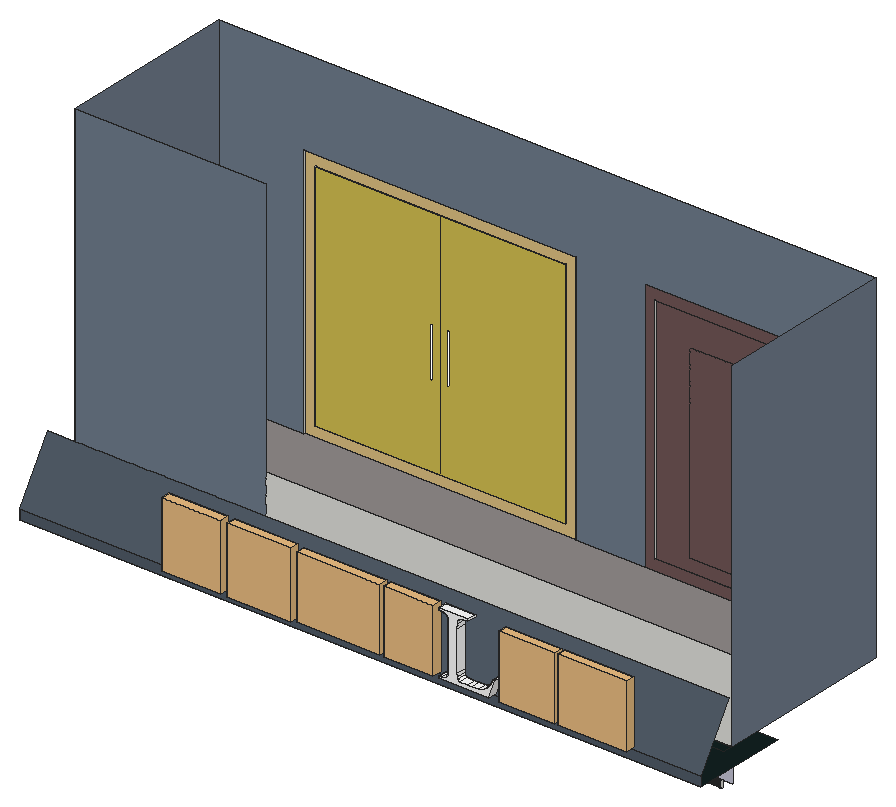
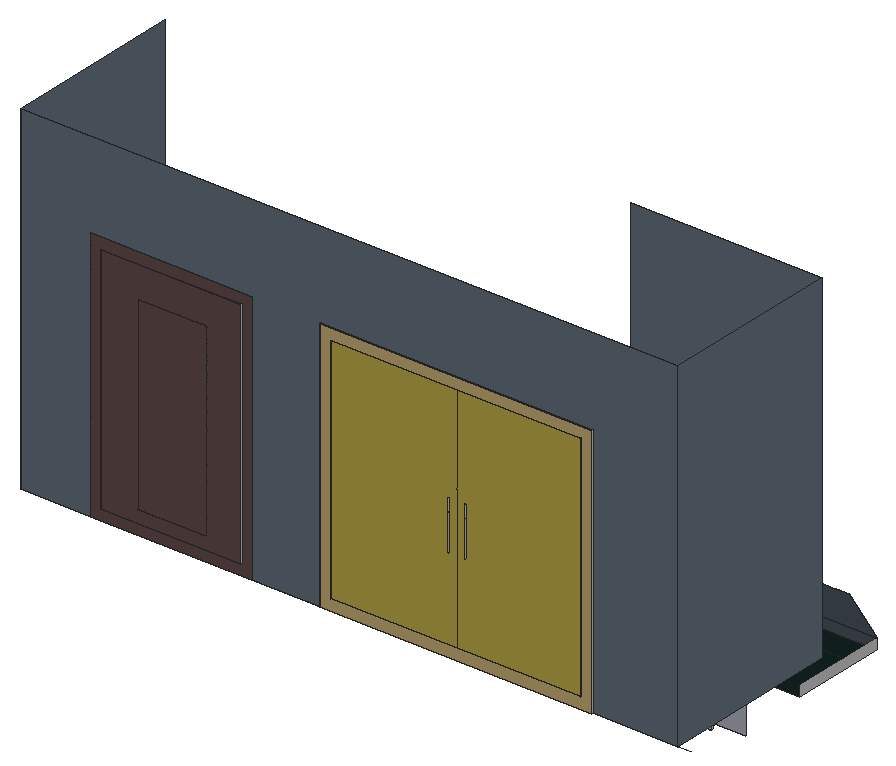
# SketchUp Ruby script. Lengths in millimetres.
U = 1.mm
M = Sketchup.active_model
def pt(a) = Geom::Point3d.new(a.map { |v| v * U })
def face(e, loops, mat)
  f = e.add_face(loops[0].map { |a| pt(a) })
  loops[1..].each { |l| e.add_face(l.map { |a| pt(a) }).erase! }
  f.material = f.back_material = mat if mat
  f
end
# faces: each face lists its corners as indices into pts; further lists are holes
def faces(e, pts, list, mat = nil) = list.each { |f| face(e, (f[0].is_a?(Array) ? f : [f]).map { |l| l.map { |i| pts[i] } }, mat) }
# xy, xz, yz: faces in a plane at the given z, y or x. An outline is a flat list of corners, or four numbers for a rectangle; further outlines are holes
def ring(l) = l.size == 4 ? [[l[0], l[1]], [l[2], l[1]], [l[2], l[3]], [l[0], l[3]]] : l.each_slice(2).to_a
def flat(e, list, mat, &to3) = list.each { |f| face(e, (f[0].is_a?(Array) ? f : [f]).map { |l| ring(l).map { |u, v| to3.(u, v) } }, mat) }
def xy(e, z, list, mat = nil) = flat(e, list, mat) { |x, y| [x, y, z] }
def xz(e, y, list, mat = nil) = flat(e, list, mat) { |x, z| [x, y, z] }
def yz(e, x, list, mat = nil) = flat(e, list, mat) { |y, z| [x, y, z] }
def lines(e, pts, list) = list.each { |a, b| e.add_line(pt(pts[a]), pt(pts[b])) }
# prism: a flat outline (further loops are holes) pulled along v
def prism(e, loops, v, mat = nil)
  f = face(e, loops, mat); d = Geom::Vector3d.new(v.map { |x| x * U })
  f.pushpull(f.normal.samedirection?(d) ? d.length : -d.length)
end
def box(e, o, s, mat = nil) = prism(e, [[o, [o[0] + s[0], o[1], o[2]], [o[0] + s[0], o[1] + s[1], o[2]], [o[0], o[1] + s[1], o[2]]]], [0, 0, s[2]], mat)
def at(x, y, z, deg = 0) = Geom::Transformation.translation(pt([x, y, z])) * Geom::Transformation.rotation(ORIGIN, Z_AXIS, deg.degrees)
def axes(o, x, y, z) = Geom::Transformation.new([*x, 0, *y, 0, *z, 0, *pt(o).to_a, 1])
def part(name) = M.definitions.add(name)
# library, detail: a bought-in or finely detailed component or shape, given as its bounding box
def library(name, o, s) = part(name).tap { |d| box(d.entities, o, s) }
def detail(e, o, s) = box(e.add_group.entities, o, s)
def put(e, d, t, mat = nil) = e.add_instance(d, t).tap { |i| i.material = mat if mat }
def group(e, t, mat = nil) = e.add_group.tap { |g| g.transformation = t; g.material = mat if mat }.entities
root = M.entities
M.materials.add("[0078_DarkSlateGray]").color = [19, 33, 33]
M.materials.add("[0099_LightSteelBlue]").color = [113, 126, 142]
M.materials.add("[0111_SlateGray]").color = [81, 92, 104]
M.materials.add("[0116_Lavender]").color = [197, 197, 214]
M.materials.add("[0119_RosyBrown]").color = [114, 87, 87]
M.materials.add("[0128_White]1").color = [255, 255, 255]
M.materials.add("[0130_Gainsboro]").color = [220, 220, 220]
M.materials.add("[Checker Plate]").color = [214, 195, 82]
M.materials.add("[Stone Brushed Khaki]").color = [226, 197, 133]
M.materials.add("[Stone Marble]").color = [143, 138, 136]
c1 = part("COMPLEX")
prism(c1.entities,[[[14980.3,871.5,0],[15051.1,856.4,0],[14802.1,66.5,0],[12548.3,66.5,0],[12548.3,146,0],[12657.8,146,0],[12816.1,176,0],[12921.8,266.2,0],[12955.6,379.9,0],[12966.9,583.8,0],[12966.9,2462,0],[12951.9,2683.6,0],[12906.8,2803.3,0],[12802.7,2874.1,0],[12657.8,2897.7,0],[12548.3,2897.7,0],[12548.3,2977.2,0],[13866.3,2977.2,0],[13866.3,2897.7,0],[13669,2888.1,0],[13541.1,2854.8,0],[13462.4,2803.8,0],[13413.3,2741.1,0],[13387.6,2624.6,0],[13379,2412.6,0],[13379,583.8,0],[13387.6,433.6,0],[13413.3,339.1,0],[13492.8,272.6,0],[13827.6,251.1,0],[14040.1,251.1,0],[14325.1,263.5,0],[14510.2,300.5,0],[14639.5,368.9,0],[14757,475.4,0],[14868.7,637.2,0]]],[0,0,406.4])
detail(c1.entities,[158.8,0,0],[2620.9,3043.7,406.4])
detail(c1.entities,[3086.6,0,0],[2850.6,3043.7,406.4])
detail(c1.entities,[6179.7,66.5,0],[3743.5,2910.7,406.4])
detail(c1.entities,[10088.5,66.5,0],[2217.3,2910.7,406.4])
detail(c1.entities,[15235.7,66.5,0],[2494.2,2910.7,406.4])
detail(c1.entities,[17863,66.5,0],[3090.9,2910.7,406.4])
xy(root,17541.9,[[9201.9,13957.3,9154.1,13959.8,9106.8,13967.3,9060.6,13979.7,9015.9,13996.8,8973.3,14018.6,8933.1,14044.6,8895.9,14074.7,8862.1,14108.6,8832,14145.8,8805.9,14185.9,8784.2,14228.5,8767.1,14273.2,8754.7,14319.4,8747.2,14366.7,8744.7,14414.5,8747.2,14462.3,8754.7,14509.6,8767.1,14555.8,8784.2,14600.5,8805.9,14643.1,8832,14683.2,8862.1,14720.4,8895.9,14754.3,8933.1,14784.4,8973.3,14810.4,9015.9,14832.2,9060.6,14849.3,9106.8,14861.7,9154.1,14869.2,9201.9,14871.7,9249.7,14869.2,9296.9,14861.7,9343.2,14849.3,9387.8,14832.2,9430.5,14810.4,9470.6,14784.4,9507.8,14754.3,9541.6,14720.4,9571.8,14683.2,9597.8,14643.1,9619.5,14600.5,9636.7,14555.8,9649.1,14509.6,9656.6,14462.3,9659.1,14414.5,9656.6,14366.7,9649.1,14319.4,9636.7,14273.2,9619.5,14228.5,9597.8,14185.9,9571.8,14145.8,9541.6,14108.6,9507.8,14074.7,9470.6,14044.6,9430.5,14018.6,9387.8,13996.8,9343.2,13979.7,9296.9,13967.3,9249.7,13959.8],[15297.9,13957.3,15250.1,13959.8,15202.8,13967.3,15156.6,13979.7,15111.9,13996.8,15069.3,14018.6,15029.1,14044.6,14991.9,14074.7,14958.1,14108.6,14928,14145.8,14901.9,14185.9,14880.2,14228.5,14863.1,14273.2,14850.7,14319.4,14843.2,14366.7,14840.7,14414.5,14843.2,14462.3,14850.7,14509.6,14863.1,14555.8,14880.2,14600.5,14901.9,14643.1,14928,14683.2,14958.1,14720.4,14991.9,14754.3,15029.1,14784.4,15069.3,14810.4,15111.9,14832.2,15156.6,14849.3,15202.8,14861.7,15250.1,14869.2,15297.9,14871.7,15345.7,14869.2,15392.9,14861.7,15439.2,14849.3,15483.8,14832.2,15526.5,14810.4,15566.6,14784.4,15603.8,14754.3,15637.6,14720.4,15667.8,14683.2,15693.8,14643.1,15715.5,14600.5,15732.7,14555.8,15745.1,14509.6,15752.6,14462.3,15755.1,14414.5,15752.6,14366.7,15745.1,14319.4,15732.7,14273.2,15715.5,14228.5,15693.8,14185.9,15667.8,14145.8,15637.6,14108.6,15603.8,14074.7,15566.6,14044.6,15526.5,14018.6,15483.8,13996.8,15439.2,13979.7,15392.9,13967.3,15345.7,13959.8],[21393.9,13957.3,21346.1,13959.8,21298.8,13967.3,21252.6,13979.7,21207.9,13996.8,21165.3,14018.6,21125.1,14044.6,21087.9,14074.7,21054.1,14108.6,21024,14145.8,20997.9,14185.9,20976.2,14228.5,20959.1,14273.2,20946.7,14319.4,20939.2,14366.7,20936.7,14414.5,20939.2,14462.3,20946.7,14509.6,20959.1,14555.8,20976.2,14600.5,20997.9,14643.1,21024,14683.2,21054.1,14720.4,21087.9,14754.3,21125.1,14784.4,21165.3,14810.4,21207.9,14832.2,21252.6,14849.3,21298.8,14861.7,21346.1,14869.2,21393.9,14871.7,21441.7,14869.2,21488.9,14861.7,21535.2,14849.3,21579.8,14832.2,21622.5,14810.4,21662.6,14784.4,21699.8,14754.3,21733.6,14720.4,21763.8,14683.2,21789.8,14643.1,21811.5,14600.5,21828.7,14555.8,21841.1,14509.6,21848.6,14462.3,21851.1,14414.5,21848.6,14366.7,21841.1,14319.4,21828.7,14273.2,21811.5,14228.5,21789.8,14185.9,21763.8,14145.8,21733.6,14108.6,21699.8,14074.7,21662.6,14044.6,21622.5,14018.6,21579.8,13996.8,21535.2,13979.7,21488.9,13967.3,21441.7,13959.8],[27489.9,13957.3,27442.1,13959.8,27394.8,13967.3,27348.6,13979.7,27303.9,13996.8,27261.3,14018.6,27221.1,14044.6,27183.9,14074.7,27150.1,14108.6,27120,14145.8,27093.9,14185.9,27072.2,14228.5,27055.1,14273.2,27042.7,14319.4,27035.2,14366.7,27032.7,14414.5,27035.2,14462.3,27042.7,14509.6,27055.1,14555.8,27072.2,14600.5,27093.9,14643.1,27120,14683.2,27150.1,14720.4,27183.9,14754.3,27221.1,14784.4,27261.3,14810.4,27303.9,14832.2,27348.6,14849.3,27394.8,14861.7,27442.1,14869.2,27489.9,14871.7,27537.7,14869.2,27584.9,14861.7,27631.2,14849.3,27675.8,14832.2,27718.5,14810.4,27758.6,14784.4,27795.8,14754.3,27829.6,14720.4,27859.8,14683.2,27885.8,14643.1,27907.5,14600.5,27924.7,14555.8,27937.1,14509.6,27944.6,14462.3,27947.1,14414.5,27944.6,14366.7,27937.1,14319.4,27924.7,14273.2,27907.5,14228.5,27885.8,14185.9,27859.8,14145.8,27829.6,14108.6,27795.8,14074.7,27758.6,14044.6,27718.5,14018.6,27675.8,13996.8,27631.2,13979.7,27584.9,13967.3,27537.7,13959.8],[33585.9,13957.3,33538.1,13959.8,33490.8,13967.3,33444.6,13979.7,33399.9,13996.8,33357.3,14018.6,33317.1,14044.6,33279.9,14074.7,33246.1,14108.6,33216,14145.8,33189.9,14185.9,33168.2,14228.5,33151.1,14273.2,33138.7,14319.4,33131.2,14366.7,33128.7,14414.5,33131.2,14462.3,33138.7,14509.6,33151.1,14555.8,33168.2,14600.5,33189.9,14643.1,33216,14683.2,33246.1,14720.4,33279.9,14754.3,33317.1,14784.4,33357.3,14810.4,33399.9,14832.2,33444.6,14849.3,33490.8,14861.7,33538.1,14869.2,33585.9,14871.7,33633.7,14869.2,33680.9,14861.7,33727.2,14849.3,33771.8,14832.2,33814.5,14810.4,33854.6,14784.4,33891.8,14754.3,33925.6,14720.4,33955.8,14683.2,33981.8,14643.1,34003.5,14600.5,34020.7,14555.8,34033.1,14509.6,34040.6,14462.3,34043.1,14414.5,34040.6,14366.7,34033.1,14319.4,34020.7,14273.2,34003.5,14228.5,33981.8,14185.9,33955.8,14145.8,33925.6,14108.6,33891.8,14074.7,33854.6,14044.6,33814.5,14018.6,33771.8,13996.8,33727.2,13979.7,33680.9,13967.3,33633.7,13959.8]])
xy(root,17541.9,[[[7076.1,12280.9,37556.1,16548.1],[9201.9,13957.3,9249.7,13959.8,9296.9,13967.3,9343.2,13979.7,9387.8,13996.8,9430.5,14018.6,9470.6,14044.6,9507.8,14074.7,9541.6,14108.6,9571.8,14145.8,9597.8,14185.9,9619.5,14228.5,9636.7,14273.2,9649.1,14319.4,9656.6,14366.7,9659.1,14414.5,9656.6,14462.3,9649.1,14509.6,9636.7,14555.8,9619.5,14600.5,9597.8,14643.1,9571.8,14683.2,9541.6,14720.4,9507.8,14754.3,9470.6,14784.4,9430.5,14810.4,9387.8,14832.2,9343.2,14849.3,9296.9,14861.7,9249.7,14869.2,9201.9,14871.7,9154.1,14869.2,9106.8,14861.7,9060.6,14849.3,9015.9,14832.2,8973.3,14810.4,8933.1,14784.4,8895.9,14754.3,8862.1,14720.4,8832,14683.2,8805.9,14643.1,8784.2,14600.5,8767.1,14555.8,8754.7,14509.6,8747.2,14462.3,8744.7,14414.5,8747.2,14366.7,8754.7,14319.4,8767.1,14273.2,8784.2,14228.5,8805.9,14185.9,8832,14145.8,8862.1,14108.6,8895.9,14074.7,8933.1,14044.6,8973.3,14018.6,9015.9,13996.8,9060.6,13979.7,9106.8,13967.3,9154.1,13959.8],[21393.9,13957.3,21441.7,13959.8,21488.9,13967.3,21535.2,13979.7,21579.8,13996.8,21622.5,14018.6,21662.6,14044.6,21699.8,14074.7,21733.6,14108.6,21763.8,14145.8,21789.8,14185.9,21811.5,14228.5,21828.7,14273.2,21841.1,14319.4,21848.6,14366.7,21851.1,14414.5,21848.6,14462.3,21841.1,14509.6,21828.7,14555.8,21811.5,14600.5,21789.8,14643.1,21763.8,14683.2,21733.6,14720.4,21699.8,14754.3,21662.6,14784.4,21622.5,14810.4,21579.8,14832.2,21535.2,14849.3,21488.9,14861.7,21441.7,14869.2,21393.9,14871.7,21346.1,14869.2,21298.8,14861.7,21252.6,14849.3,21207.9,14832.2,21165.3,14810.4,21125.1,14784.4,21087.9,14754.3,21054.1,14720.4,21024,14683.2,20997.9,14643.1,20976.2,14600.5,20959.1,14555.8,20946.7,14509.6,20939.2,14462.3,20936.7,14414.5,20939.2,14366.7,20946.7,14319.4,20959.1,14273.2,20976.2,14228.5,20997.9,14185.9,21024,14145.8,21054.1,14108.6,21087.9,14074.7,21125.1,14044.6,21165.3,14018.6,21207.9,13996.8,21252.6,13979.7,21298.8,13967.3,21346.1,13959.8],[15297.9,13957.3,15345.7,13959.8,15392.9,13967.3,15439.2,13979.7,15483.8,13996.8,15526.5,14018.6,15566.6,14044.6,15603.8,14074.7,15637.6,14108.6,15667.8,14145.8,15693.8,14185.9,15715.5,14228.5,15732.7,14273.2,15745.1,14319.4,15752.6,14366.7,15755.1,14414.5,15752.6,14462.3,15745.1,14509.6,15732.7,14555.8,15715.5,14600.5,15693.8,14643.1,15667.8,14683.2,15637.6,14720.4,15603.8,14754.3,15566.6,14784.4,15526.5,14810.4,15483.8,14832.2,15439.2,14849.3,15392.9,14861.7,15345.7,14869.2,15297.9,14871.7,15250.1,14869.2,15202.8,14861.7,15156.6,14849.3,15111.9,14832.2,15069.3,14810.4,15029.1,14784.4,14991.9,14754.3,14958.1,14720.4,14928,14683.2,14901.9,14643.1,14880.2,14600.5,14863.1,14555.8,14850.7,14509.6,14843.2,14462.3,14840.7,14414.5,14843.2,14366.7,14850.7,14319.4,14863.1,14273.2,14880.2,14228.5,14901.9,14185.9,14928,14145.8,14958.1,14108.6,14991.9,14074.7,15029.1,14044.6,15069.3,14018.6,15111.9,13996.8,15156.6,13979.7,15202.8,13967.3,15250.1,13959.8],[33585.9,13957.3,33633.7,13959.8,33680.9,13967.3,33727.2,13979.7,33771.8,13996.8,33814.5,14018.6,33854.6,14044.6,33891.8,14074.7,33925.6,14108.6,33955.8,14145.8,33981.8,14185.9,34003.5,14228.5,34020.7,14273.2,34033.1,14319.4,34040.6,14366.7,34043.1,14414.5,34040.6,14462.3,34033.1,14509.6,34020.7,14555.8,34003.5,14600.5,33981.8,14643.1,33955.8,14683.2,33925.6,14720.4,33891.8,14754.3,33854.6,14784.4,33814.5,14810.4,33771.8,14832.2,33727.2,14849.3,33680.9,14861.7,33633.7,14869.2,33585.9,14871.7,33538.1,14869.2,33490.8,14861.7,33444.6,14849.3,33399.9,14832.2,33357.3,14810.4,33317.1,14784.4,33279.9,14754.3,33246.1,14720.4,33216,14683.2,33189.9,14643.1,33168.2,14600.5,33151.1,14555.8,33138.7,14509.6,33131.2,14462.3,33128.7,14414.5,33131.2,14366.7,33138.7,14319.4,33151.1,14273.2,33168.2,14228.5,33189.9,14185.9,33216,14145.8,33246.1,14108.6,33279.9,14074.7,33317.1,14044.6,33357.3,14018.6,33399.9,13996.8,33444.6,13979.7,33490.8,13967.3,33538.1,13959.8],[27489.9,13957.3,27537.7,13959.8,27584.9,13967.3,27631.2,13979.7,27675.8,13996.8,27718.5,14018.6,27758.6,14044.6,27795.8,14074.7,27829.6,14108.6,27859.8,14145.8,27885.8,14185.9,27907.5,14228.5,27924.7,14273.2,27937.1,14319.4,27944.6,14366.7,27947.1,14414.5,27944.6,14462.3,27937.1,14509.6,27924.7,14555.8,27907.5,14600.5,27885.8,14643.1,27859.8,14683.2,27829.6,14720.4,27795.8,14754.3,27758.6,14784.4,27718.5,14810.4,27675.8,14832.2,27631.2,14849.3,27584.9,14861.7,27537.7,14869.2,27489.9,14871.7,27442.1,14869.2,27394.8,14861.7,27348.6,14849.3,27303.9,14832.2,27261.3,14810.4,27221.1,14784.4,27183.9,14754.3,27150.1,14720.4,27120,14683.2,27093.9,14643.1,27072.2,14600.5,27055.1,14555.8,27042.7,14509.6,27035.2,14462.3,27032.7,14414.5,27035.2,14366.7,27042.7,14319.4,27055.1,14273.2,27072.2,14228.5,27093.9,14185.9,27120,14145.8,27150.1,14108.6,27183.9,14074.7,27221.1,14044.6,27261.3,14018.6,27303.9,13996.8,27348.6,13979.7,27394.8,13967.3,27442.1,13959.8]]],"[0078_DarkSlateGray]")
xy(root,17999.1,[[7685.7,14566.9,37098.9,14566.9,37098.9,22644.1,23669.6,22644.1,23669.6,22694.9,11477.6,22694.9,11477.6,22644.1,7685.7,22644.1]],"[Stone Marble]")
xy(root,18486.8,[[11965.2,22644.1,17573.6,22694.9],[17573.6,22644.1,23181.9,22694.9],[27205.2,22644.1,33459.3,22694.9]])
xz(root,12280.9,[[7076.1,17541.9,37556.1,17999.1]],"[0111_SlateGray]")
xz(root,14566.9,[[16220.1,17999.1,37098.9,21656.7]])
xz(root,14566.9,[[7685.7,17999.1,16220.1,33239.1]],"[0099_LightSteelBlue]")
xz(root,16548.1,[[11038.5,14798.7,25059.3,15103.5],[29021.7,14798.7,35117.7,15103.5]])
xz(root,16548.1,[[9514.5,15103.5,26583.3,17541.9],[28564.5,15103.5,35574.9,17541.9]],"[0116_Lavender]")
xz(root,22644.1,[[7685.7,17999.1,11477.6,17999.1,11477.6,29360.8,23669.6,29360.8,23669.6,17999.1,26717.6,17999.1,26717.6,29360.8,33947,29360.8,33947,17999.1,37098.9,17999.1,37098.9,33239.1,7685.7,33239.1]],"[0099_LightSteelBlue]")
xz(root,22644.1,[[[26717.6,17999.1,33947,29360.8],[27205.2,18486.8,33459.3,28873.1]]],"[0119_RosyBrown]")
xz(root,22644.1,[[[11965.2,18486.8,17573.6,28873.1],[17116.4,22141.2,17268.8,24406.5]],[[17573.6,18486.8,23181.9,28873.1],[17878.4,22141.2,18030.8,24406.5]]],"[Checker Plate]")
xz(root,22694.9,[[[27205.2,18486.8,33459.3,28873.1],[28719.8,19052.1,31788.4,27486.5]],[28719.8,19052.1,31788.4,27486.5]],"[0119_RosyBrown]")
xz(root,22694.9,[[[11477.6,17999.1,23669.6,29360.8],[11965.2,18486.8,23181.9,28873.1]]],"[Stone Brushed Khaki]")
yz(root,7076.1,[[12280.9,17541.9,16548.1,17999.1]],"[0130_Gainsboro]")
yz(root,7685.7,[[14566.9,17999.1,22644.1,33239.1]],"[0099_LightSteelBlue]")
yz(root,11038.5,[[16548.1,14798.7,16536.2,14804,16524.8,14810.3,16514,14817.4,16503.7,14825.4,16494.1,14834.2,16485.2,14843.7,16477.1,14853.8,16469.8,14864.6,16463.4,14875.9,16458,14887.7,16453.4,14899.9,16449.9,14912.4,16447.3,14925.2,16445.8,14938.1,16445.3,14951.1,16445.8,14964.1,16447.3,14977,16449.9,14989.7,16453.4,15002.2,16458,15014.4,16463.4,15026.2,16469.8,15037.5,16477.1,15048.3,16485.2,15058.5,16494.1,15068,16503.7,15076.8,16514,15084.7,16524.8,15091.9,16536.2,15098.1,16548.1,15103.5]])
yz(root,11477.6,[[22644.1,17999.1,22694.9,29360.8]])
yz(root,11965.2,[[22644.1,18486.8,22694.9,28873.1]])
yz(root,23181.9,[[22644.1,18486.8,22694.9,28873.1]])
yz(root,23669.6,[[22644.1,17999.1,22694.9,29360.8]])
yz(root,25059.3,[[16548.1,14798.7,16548.1,15103.5,16536.2,15098.1,16524.8,15091.9,16514,15084.7,16503.7,15076.8,16494.1,15068,16485.2,15058.5,16477.1,15048.3,16469.8,15037.5,16463.4,15026.2,16458,15014.4,16453.4,15002.2,16449.9,14989.7,16447.3,14977,16445.8,14964.1,16445.3,14951.1,16445.8,14938.1,16447.3,14925.2,16449.9,14912.4,16453.4,14899.9,16458,14887.7,16463.4,14875.9,16469.8,14864.6,16477.1,14853.8,16485.2,14843.7,16494.1,14834.2,16503.7,14825.4,16514,14817.4,16524.8,14810.3,16536.2,14804]])
yz(root,27205.2,[[22644.1,18486.8,22694.9,28873.1]])
yz(root,29021.7,[[16548.1,14798.7,16540.1,14798.9,16532.2,14799.5,16524.3,14800.6,16516.4,14802,16508.7,14803.9,16501,14806.1,16493.5,14808.8,16486.1,14811.9,16478.9,14815.3,16471.9,14819.1,16465.1,14823.3,16458.5,14827.8,16452.2,14832.6,16446.1,14837.8,16440.3,14843.3,16434.8,14849.1,16429.7,14855.2,16424.8,14861.5,16420.3,14868.1,16416.1,14874.9,16412.3,14881.9,16408.9,14889.1,16405.8,14896.5,16403.2,14904,16400.9,14911.6,16399,14919.4,16397.6,14927.2,16396.5,14935.1,16395.9,14943.1,16395.7,14951.1,16395.9,14959.1,16396.5,14967,16397.6,14974.9,16399,14982.8,16400.9,14990.5,16403.2,14998.2,16405.8,15005.7,16408.9,15013.1,16412.3,15020.3,16416.1,15027.3,16420.3,15034.1,16424.8,15040.7,16429.7,15047,16434.8,15053.1,16440.3,15058.8,16446.1,15064.3,16452.2,15069.5,16458.5,15074.4,16465.1,15078.9,16471.9,15083.1,16478.9,15086.9,16486.1,15090.3,16493.5,15093.4,16501,15096,16508.7,15098.3,16516.4,15100.1,16524.3,15101.6,16532.2,15102.6,16540.1,15103.3,16548.1,15103.5]])
yz(root,33459.3,[[22644.1,18486.8,22694.9,28873.1]])
yz(root,35117.7,[[16548.1,14798.7,16548.1,15103.5,16540.1,15103.3,16532.2,15102.6,16524.3,15101.6,16516.4,15100.1,16508.7,15098.3,16501,15096,16493.5,15093.4,16486.1,15090.3,16478.9,15086.9,16471.9,15083.1,16465.1,15078.9,16458.5,15074.4,16452.2,15069.5,16446.1,15064.3,16440.3,15058.8,16434.8,15053.1,16429.7,15047,16424.8,15040.7,16420.3,15034.1,16416.1,15027.3,16412.3,15020.3,16408.9,15013.1,16405.8,15005.7,16403.2,14998.2,16400.9,14990.5,16399,14982.8,16397.6,14974.9,16396.5,14967,16395.9,14959.1,16395.7,14951.1,16395.9,14943.1,16396.5,14935.1,16397.6,14927.2,16399,14919.4,16400.9,14911.6,16403.2,14904,16405.8,14896.5,16408.9,14889.1,16412.3,14881.9,16416.1,14874.9,16420.3,14868.1,16424.8,14861.5,16429.7,14855.2,16434.8,14849.1,16440.3,14843.3,16446.1,14837.8,16452.2,14832.6,16458.5,14827.8,16465.1,14823.3,16471.9,14819.1,16478.9,14815.3,16486.1,14811.9,16493.5,14808.8,16501,14806.1,16508.7,14803.9,16516.4,14802,16524.3,14800.6,16532.2,14799.5,16540.1,14798.9]])
yz(root,37098.9,[[14566.9,17999.1,22644.1,33239.1]],"[0099_LightSteelBlue]")
p = [[25059.3,16548.1,14798.7],[25059.3,16536.2,14804],[11038.5,16536.2,14804],[11038.5,16548.1,14798.7],[35117.7,16548.1,14798.7],[35117.7,16540.1,14798.9],
  [29021.7,16540.1,14798.9],[29021.7,16548.1,14798.7],[35117.7,16532.2,14799.5],[29021.7,16532.2,14799.5],[35117.7,16524.3,14800.6],[29021.7,16524.3,14800.6],
  [35117.7,16516.4,14802],[29021.7,16516.4,14802],[35117.7,16508.7,14803.9],[29021.7,16508.7,14803.9],[35117.7,16501,14806.1],[29021.7,16501,14806.1],
  [25059.3,16524.8,14810.3],[11038.5,16524.8,14810.3],[35117.7,16493.5,14808.8],[29021.7,16493.5,14808.8],[35117.7,16486.1,14811.9],[29021.7,16486.1,14811.9],
  [25059.3,16514,14817.4],[11038.5,16514,14817.4],[35117.7,16478.9,14815.3],[29021.7,16478.9,14815.3],[35117.7,16471.9,14819.1],[29021.7,16471.9,14819.1],
  [25059.3,16503.7,14825.4],[11038.5,16503.7,14825.4],[35117.7,16465.1,14823.3],[29021.7,16465.1,14823.3],[35117.7,16458.5,14827.8],[29021.7,16458.5,14827.8],
  [25059.3,16494.1,14834.2],[11038.5,16494.1,14834.2],[35117.7,16452.2,14832.6],[29021.7,16452.2,14832.6],[35117.7,16446.1,14837.8],[29021.7,16446.1,14837.8],
  [25059.3,16485.2,14843.7],[11038.5,16485.2,14843.7],[35117.7,16440.3,14843.3],[29021.7,16440.3,14843.3],[35117.7,16434.8,14849.1],[29021.7,16434.8,14849.1],
  [25059.3,16477.1,14853.8],[11038.5,16477.1,14853.8],[35117.7,16429.7,14855.2],[29021.7,16429.7,14855.2],[25059.3,16469.8,14864.6],[11038.5,16469.8,14864.6],
  [35117.7,16424.8,14861.5],[29021.7,16424.8,14861.5],[35117.7,16420.3,14868.1],[29021.7,16420.3,14868.1],[25059.3,16463.4,14875.9],[11038.5,16463.4,14875.9],
  [35117.7,16416.1,14874.9],[29021.7,16416.1,14874.9],[35117.7,16412.3,14881.9],[29021.7,16412.3,14881.9],[25059.3,16458,14887.7],[11038.5,16458,14887.7],
  [35117.7,16408.9,14889.1],[29021.7,16408.9,14889.1],[25059.3,16453.4,14899.9],[11038.5,16453.4,14899.9],[35117.7,16405.8,14896.5],[29021.7,16405.8,14896.5],
  [35117.7,16403.2,14904],[29021.7,16403.2,14904],[25059.3,16449.9,14912.4],[11038.5,16449.9,14912.4],[35117.7,16400.9,14911.6],[29021.7,16400.9,14911.6],
  [35117.7,16399,14919.4],[29021.7,16399,14919.4],[25059.3,16447.3,14925.2],[11038.5,16447.3,14925.2],[35117.7,16397.6,14927.2],[29021.7,16397.6,14927.2],
  [25059.3,16445.8,14938.1],[11038.5,16445.8,14938.1],[35117.7,16396.5,14935.1],[29021.7,16396.5,14935.1],[35117.7,16395.9,14943.1],[29021.7,16395.9,14943.1],
  [25059.3,16445.3,14951.1],[11038.5,16445.3,14951.1],[35117.7,16395.7,14951.1],[29021.7,16395.7,14951.1],[35117.7,16395.9,14959.1],[29021.7,16395.9,14959.1],
  [25059.3,16445.8,14964.1],[11038.5,16445.8,14964.1],[35117.7,16396.5,14967],[29021.7,16396.5,14967],[25059.3,16447.3,14977],[11038.5,16447.3,14977],
  [35117.7,16397.6,14974.9],[29021.7,16397.6,14974.9],[35117.7,16399,14982.8],[29021.7,16399,14982.8],[25059.3,16449.9,14989.7],[11038.5,16449.9,14989.7],
  [35117.7,16400.9,14990.5],[29021.7,16400.9,14990.5],[25059.3,16453.4,15002.2],[11038.5,16453.4,15002.2],[35117.7,16403.2,14998.2],[29021.7,16403.2,14998.2],
  [35117.7,16405.8,15005.7],[29021.7,16405.8,15005.7],[25059.3,16458,15014.4],[11038.5,16458,15014.4],[35117.7,16408.9,15013.1],[29021.7,16408.9,15013.1],
  [35117.7,16412.3,15020.3],[29021.7,16412.3,15020.3],[25059.3,16463.4,15026.2],[11038.5,16463.4,15026.2],[35117.7,16416.1,15027.3],[29021.7,16416.1,15027.3],
  [25059.3,16469.8,15037.5],[11038.5,16469.8,15037.5],[35117.7,16420.3,15034.1],[29021.7,16420.3,15034.1],[35117.7,16424.8,15040.7],[29021.7,16424.8,15040.7],
  [25059.3,16477.1,15048.3],[11038.5,16477.1,15048.3],[35117.7,16429.7,15047],[29021.7,16429.7,15047],[35117.7,16434.8,15053.1],[29021.7,16434.8,15053.1],
  [25059.3,16485.2,15058.5],[11038.5,16485.2,15058.5],[35117.7,16440.3,15058.8],[29021.7,16440.3,15058.8],[25059.3,16494.1,15068],[11038.5,16494.1,15068],
  [35117.7,16446.1,15064.3],[29021.7,16446.1,15064.3],[35117.7,16452.2,15069.5],[29021.7,16452.2,15069.5],[25059.3,16503.7,15076.8],[11038.5,16503.7,15076.8],
  [35117.7,16458.5,15074.4],[29021.7,16458.5,15074.4],[35117.7,16465.1,15078.9],[29021.7,16465.1,15078.9],[25059.3,16514,15084.7],[11038.5,16514,15084.7],
  [35117.7,16471.9,15083.1],[29021.7,16471.9,15083.1],[35117.7,16478.9,15086.9],[29021.7,16478.9,15086.9],[25059.3,16524.8,15091.9],[11038.5,16524.8,15091.9],
  [35117.7,16486.1,15090.3],[29021.7,16486.1,15090.3],[35117.7,16493.5,15093.4],[29021.7,16493.5,15093.4],[25059.3,16536.2,15098.1],[11038.5,16536.2,15098.1],
  [35117.7,16501,15096],[29021.7,16501,15096],[35117.7,16508.7,15098.3],[29021.7,16508.7,15098.3],[25059.3,16548.1,15103.5],[11038.5,16548.1,15103.5],
  [35117.7,16516.4,15100.1],[29021.7,16516.4,15100.1],[35117.7,16524.3,15101.6],[29021.7,16524.3,15101.6],[35117.7,16532.2,15102.6],[29021.7,16532.2,15102.6],
  [35117.7,16540.1,15103.3],[29021.7,16540.1,15103.3],[35117.7,16548.1,15103.5],[29021.7,16548.1,15103.5],[37556.1,12280.9,17999.1],[37556.1,13804.9,20437.5],
  [16220.1,13804.9,20437.5],[15458.1,13804.9,20437.5],[15305.7,13804.9,20437.5],[14696.1,13804.9,20437.5],[14543.7,13804.9,20437.5],[13934.1,13804.9,20437.5],
  [13781.7,13804.9,20437.5],[13172.1,13804.9,20437.5],[13019.7,13804.9,20437.5],[12410.1,13804.9,20437.5],[12257.7,13804.9,20437.5],[11648.1,13804.9,20437.5],
  [11495.7,13804.9,20437.5],[10886.1,13804.9,20437.5],[10733.7,13804.9,20437.5],[10124.1,13804.9,20437.5],[9971.7,13804.9,20437.5],[9362.1,13804.9,20437.5],
  [9209.7,13804.9,20437.5],[8600.1,13804.9,20437.5],[8447.7,13804.9,20437.5],[7838.1,13804.9,20437.5],[7685.7,13804.9,20437.5],[7076.1,13804.9,20437.5],
  [7076.1,12280.9,17999.1],[7076.1,22644.1,17999.1],[7685.7,22644.1,17999.1],[37098.9,14566.9,17999.1],[37098.9,14109.7,17999.1],[7076.1,14109.7,17999.1]]
faces(root,p,[[0,1,2,3],[4,5,6,7],[5,8,9,6],[8,10,11,9],[10,12,13,11],[12,14,15,13],[14,16,17,15],[1,18,19,2],
  [16,20,21,17],[20,22,23,21],[18,24,25,19],[22,26,27,23],[26,28,29,27],[24,30,31,25],[28,32,33,29],[32,34,35,33],
  [30,36,37,31],[34,38,39,35],[38,40,41,39],[36,42,43,37],[40,44,45,41],[44,46,47,45],[42,48,49,43],[46,50,51,47],
  [48,52,53,49],[50,54,55,51],[54,56,57,55],[52,58,59,53],[56,60,61,57],[60,62,63,61],[58,64,65,59],[62,66,67,63],
  [64,68,69,65],[66,70,71,67],[70,72,73,71],[68,74,75,69],[72,76,77,73],[76,78,79,77],[74,80,81,75],[78,82,83,79],
  [80,84,85,81],[82,86,87,83],[86,88,89,87],[84,90,91,85],[88,92,93,89],[92,94,95,93],[90,96,97,91],[94,98,99,95],
  [96,100,101,97],[98,102,103,99],[102,104,105,103],[100,106,107,101],[104,108,109,105],[106,110,111,107],[108,112,113,109],[112,114,115,113],
  [110,116,117,111],[114,118,119,115],[118,120,121,119],[116,122,123,117],[120,124,125,121],[122,126,127,123],[124,128,129,125],[128,130,131,129],
  [126,132,133,127],[130,134,135,131],[134,136,137,135],[132,138,139,133],[136,140,141,137],[138,142,143,139],[140,144,145,141],[144,146,147,145],
  [142,148,149,143],[146,150,151,147],[150,152,153,151],[148,154,155,149],[152,156,157,153],[156,158,159,157],[154,160,161,155],[158,162,163,159],
  [162,164,165,163],[160,166,167,161],[164,168,169,165],[168,170,171,169],[166,172,173,167],[170,174,175,171],[174,176,177,175],[176,178,179,177],
  [178,180,181,179],[180,182,183,181]],"[0116_Lavender]")
faces(root,p,[[184,185,186,187,188,189,190,191,192,193,194,195,196,197,198,199,200,201,202,203,204,205,206,207,208,209,210]],"[0111_SlateGray]")
lines(root,p,[[211,212],[213,214],[214,215]])
put(root,c1,axes([13575,12280.9,17999.1],[1,0,0],[0,0,0.97],[0,-1,0]),"[0128_White]1")
